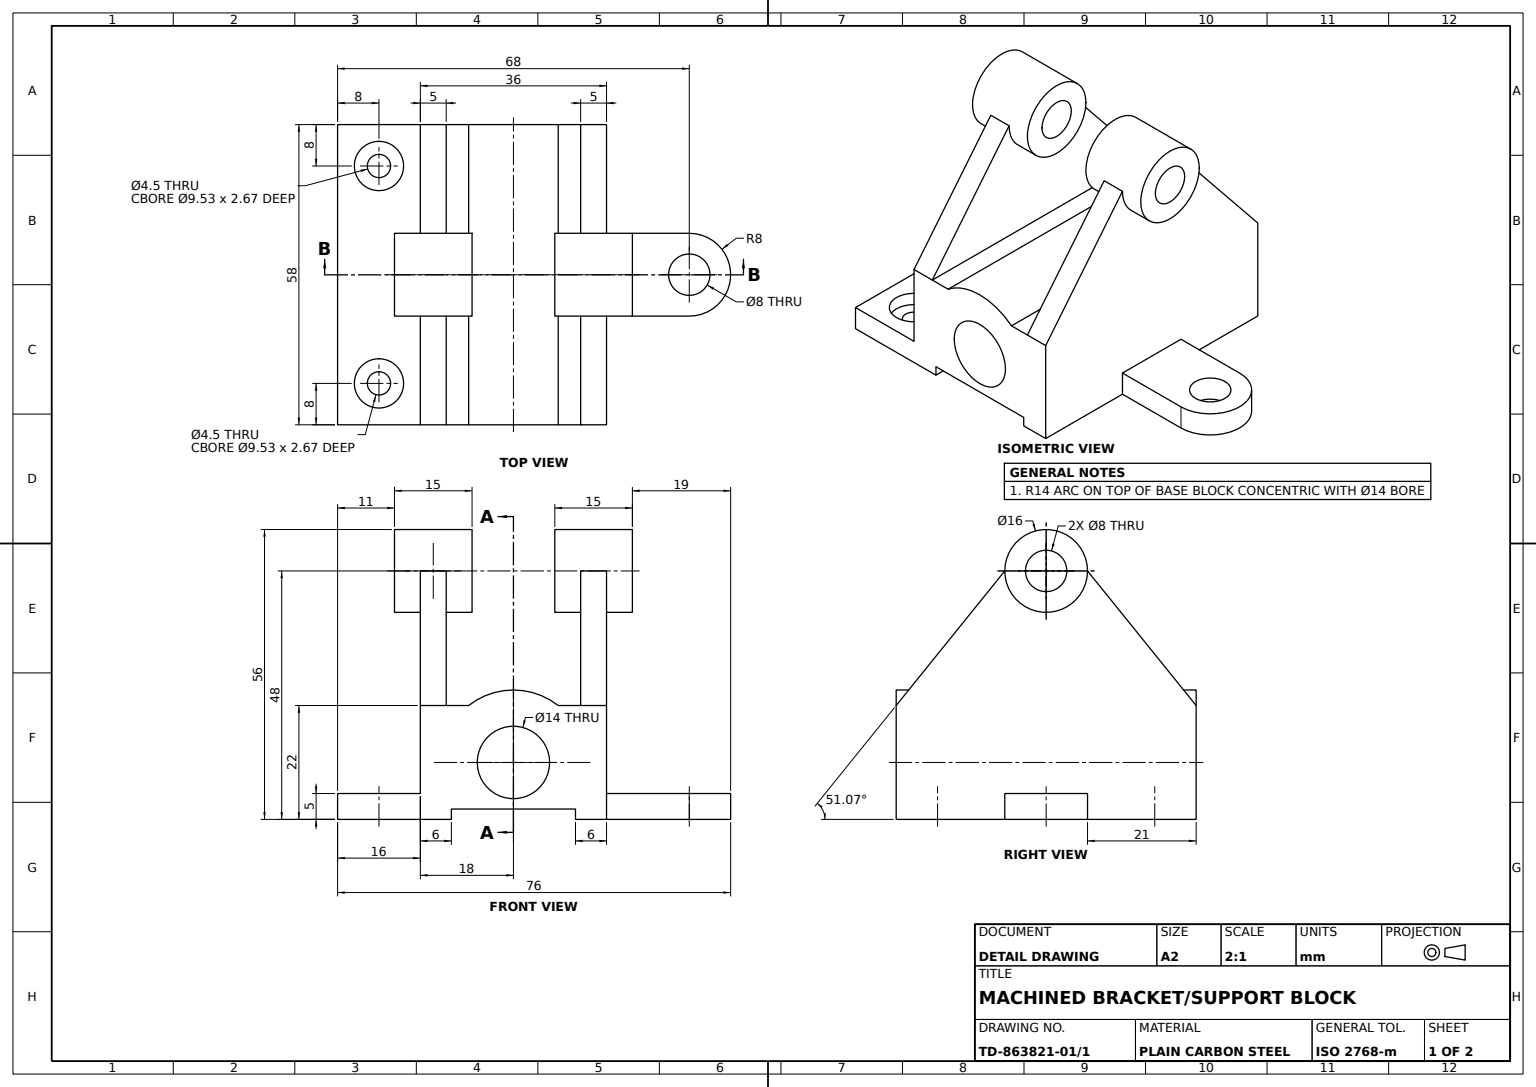
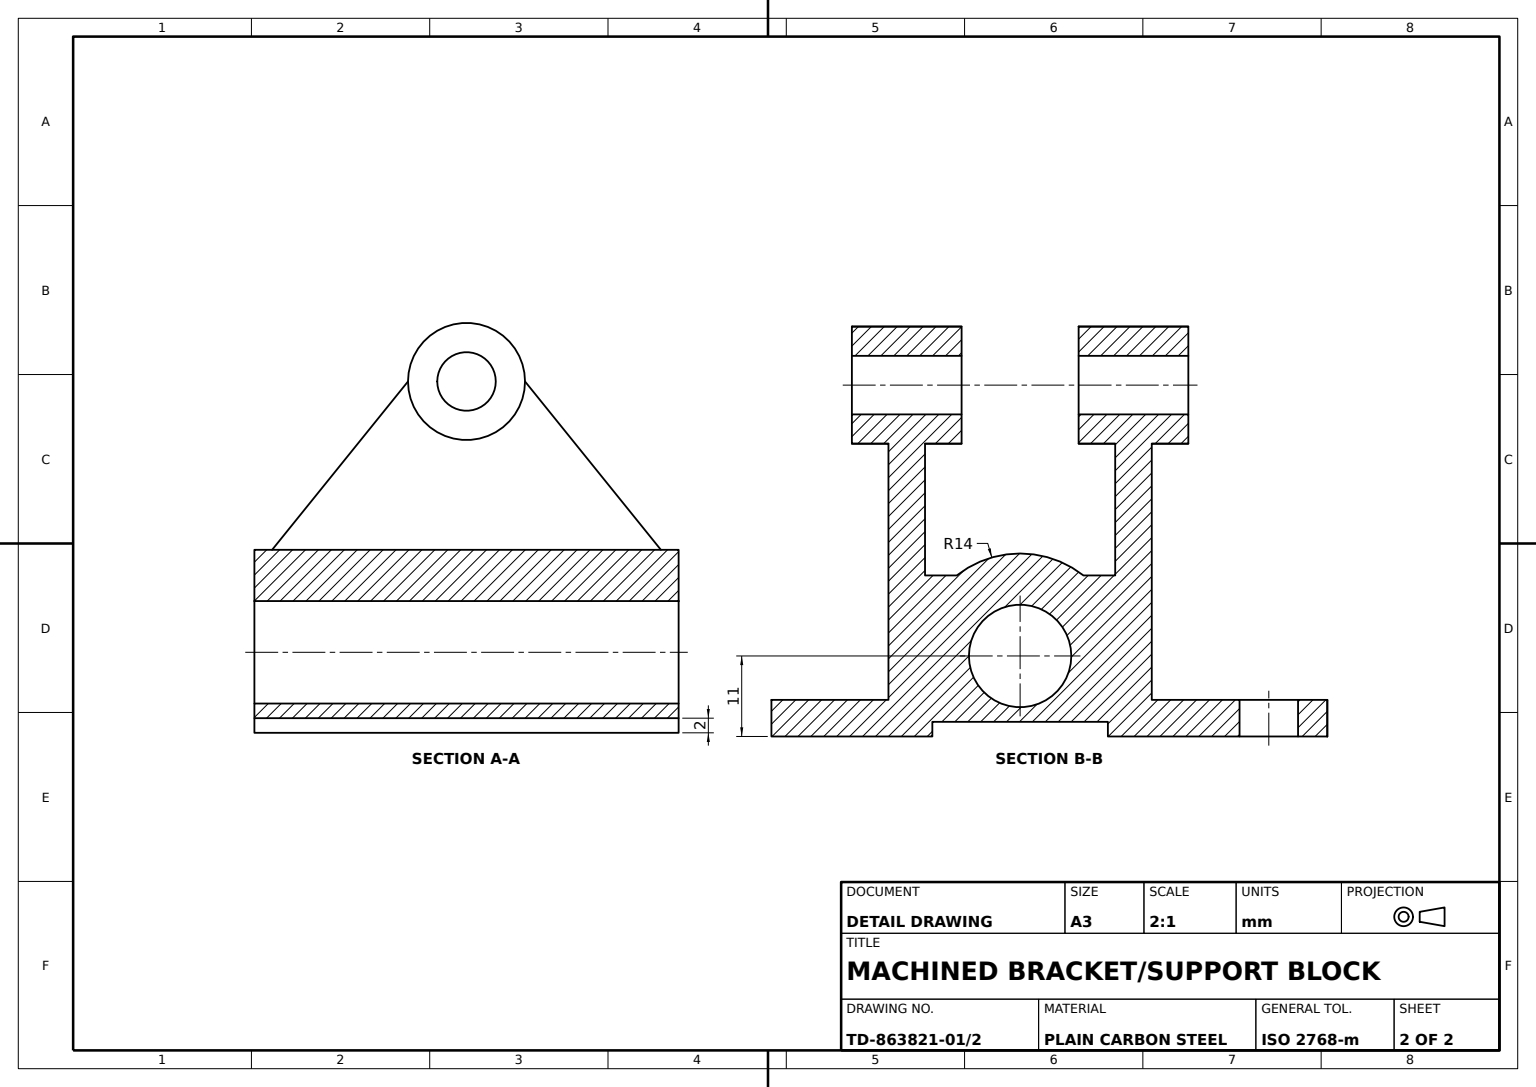
ISO-10303-21;
HEADER;
FILE_DESCRIPTION((''),'2;1');
FILE_NAME('','',(''),(''),'','','');
FILE_SCHEMA(('AUTOMOTIVE_DESIGN'));
ENDSEC;
DATA;
#1=APPLICATION_CONTEXT('');
#2=PRODUCT_CONTEXT('',#1,'mechanical');
#3=PRODUCT('','','',(#2));
#4=PRODUCT_DEFINITION_FORMATION('','',#3);
#5=PRODUCT_DEFINITION_CONTEXT('',#1,'design');
#6=PRODUCT_DEFINITION('','',#4,#5);
#7=PRODUCT_DEFINITION_SHAPE('','',#6);
#8=(LENGTH_UNIT()NAMED_UNIT(*)SI_UNIT(.MILLI.,.METRE.));
#9=(NAMED_UNIT(*)PLANE_ANGLE_UNIT()SI_UNIT($,.RADIAN.));
#10=(NAMED_UNIT(*)SI_UNIT($,.STERADIAN.)SOLID_ANGLE_UNIT());
#11=UNCERTAINTY_MEASURE_WITH_UNIT(LENGTH_MEASURE(1.E-05),#8,'distance_accuracy_value','');
#12=(GEOMETRIC_REPRESENTATION_CONTEXT(3)GLOBAL_UNCERTAINTY_ASSIGNED_CONTEXT((#11))GLOBAL_UNIT_ASSIGNED_CONTEXT((#8,#9,#10))REPRESENTATION_CONTEXT('',''));
#13=CARTESIAN_POINT('',(-8.,0.,5.75));
#14=VERTEX_POINT('',#13);
#15=CARTESIAN_POINT('',(-8.,0.,10.25));
#16=VERTEX_POINT('',#15);
#17=CARTESIAN_POINT('',(-8.,0.,8.));
#18=DIRECTION('',(0.,1.,0.));
#19=DIRECTION('',(0.,0.,1.));
#20=AXIS2_PLACEMENT_3D('',#17,#18,#19);
#21=CIRCLE('',#20,2.25);
#22=EDGE_CURVE('',#14,#16,#21,.T.);
#23=ORIENTED_EDGE('',*,*,#22,.T.);
#24=EDGE_CURVE('',#16,#14,#21,.T.);
#25=ORIENTED_EDGE('',*,*,#24,.T.);
#26=EDGE_LOOP('',(#23,#25));
#27=FACE_BOUND('',#26,.T.);
#28=CARTESIAN_POINT('',(-16.,0.,0.));
#29=VERTEX_POINT('',#28);
#30=CARTESIAN_POINT('',(6.,0.,0.));
#31=VERTEX_POINT('',#30);
#32=CARTESIAN_POINT('',(0.,0.,0.));
#33=DIRECTION('',(1.,0.,0.));
#34=VECTOR('',#33,1000.);
#35=LINE('',#32,#34);
#36=EDGE_CURVE('',#29,#31,#35,.T.);
#37=ORIENTED_EDGE('',*,*,#36,.T.);
#38=CARTESIAN_POINT('',(6.,0.,58.));
#39=VERTEX_POINT('',#38);
#40=DIRECTION('',(0.,0.,-1.));
#41=VECTOR('',#40,1000.);
#42=LINE('',#38,#41);
#43=EDGE_CURVE('',#39,#31,#42,.T.);
#44=ORIENTED_EDGE('',*,*,#43,.F.);
#45=CARTESIAN_POINT('',(-16.,0.,58.));
#46=VERTEX_POINT('',#45);
#47=CARTESIAN_POINT('',(0.,0.,58.));
#48=LINE('',#47,#34);
#49=EDGE_CURVE('',#46,#39,#48,.T.);
#50=ORIENTED_EDGE('',*,*,#49,.F.);
#51=VECTOR('',#19,1000.);
#52=LINE('',#28,#51);
#53=EDGE_CURVE('',#29,#46,#52,.T.);
#54=ORIENTED_EDGE('',*,*,#53,.F.);
#55=EDGE_LOOP('',(#37,#44,#50,#54));
#56=FACE_OUTER_BOUND('',#55,.T.);
#57=CARTESIAN_POINT('',(-8.,0.,47.75));
#58=VERTEX_POINT('',#57);
#59=CARTESIAN_POINT('',(-8.,0.,52.25));
#60=VERTEX_POINT('',#59);
#61=CARTESIAN_POINT('',(-8.,0.,50.));
#62=AXIS2_PLACEMENT_3D('',#61,#18,#19);
#63=CIRCLE('',#62,2.25);
#64=EDGE_CURVE('',#58,#60,#63,.T.);
#65=ORIENTED_EDGE('',*,*,#64,.T.);
#66=EDGE_CURVE('',#60,#58,#63,.T.);
#67=ORIENTED_EDGE('',*,*,#66,.T.);
#68=EDGE_LOOP('',(#65,#67));
#69=FACE_BOUND('',#68,.T.);
#70=AXIS2_PLACEMENT_3D('',#47,#18,#19);
#71=PLANE('',#70);
#72=ADVANCED_FACE('',(#27,#56,#69),#71,.F.);
#73=CARTESIAN_POINT('',(52.,0.,25.));
#74=VERTEX_POINT('',#73);
#75=CARTESIAN_POINT('',(52.,0.,33.));
#76=VERTEX_POINT('',#75);
#77=CARTESIAN_POINT('',(52.,0.,29.));
#78=AXIS2_PLACEMENT_3D('',#77,#18,#19);
#79=CIRCLE('',#78,4.);
#80=EDGE_CURVE('',#74,#76,#79,.T.);
#81=ORIENTED_EDGE('',*,*,#80,.T.);
#82=EDGE_CURVE('',#76,#74,#79,.T.);
#83=ORIENTED_EDGE('',*,*,#82,.T.);
#84=EDGE_LOOP('',(#81,#83));
#85=FACE_BOUND('',#84,.T.);
#86=CARTESIAN_POINT('',(36.,0.,58.));
#87=VERTEX_POINT('',#86);
#88=CARTESIAN_POINT('',(36.,0.,37.));
#89=VERTEX_POINT('',#88);
#90=LINE('',#86,#41);
#91=EDGE_CURVE('',#87,#89,#90,.T.);
#92=ORIENTED_EDGE('',*,*,#91,.F.);
#93=CARTESIAN_POINT('',(30.,0.,58.));
#94=VERTEX_POINT('',#93);
#95=LINE('',#93,#34);
#96=EDGE_CURVE('',#94,#87,#95,.T.);
#97=ORIENTED_EDGE('',*,*,#96,.F.);
#98=CARTESIAN_POINT('',(30.,0.,0.));
#99=VERTEX_POINT('',#98);
#100=LINE('',#93,#41);
#101=EDGE_CURVE('',#94,#99,#100,.T.);
#102=ORIENTED_EDGE('',*,*,#101,.T.);
#103=CARTESIAN_POINT('',(36.,0.,0.));
#104=VERTEX_POINT('',#103);
#105=LINE('',#98,#34);
#106=EDGE_CURVE('',#99,#104,#105,.T.);
#107=ORIENTED_EDGE('',*,*,#106,.T.);
#108=CARTESIAN_POINT('',(36.,0.,21.));
#109=VERTEX_POINT('',#108);
#110=EDGE_CURVE('',#109,#104,#90,.T.);
#111=ORIENTED_EDGE('',*,*,#110,.F.);
#112=CARTESIAN_POINT('',(52.,0.,21.));
#113=VERTEX_POINT('',#112);
#114=DIRECTION('',(-1.,0.,0.));
#115=VECTOR('',#114,1000.);
#116=LINE('',#112,#115);
#117=EDGE_CURVE('',#113,#109,#116,.T.);
#118=ORIENTED_EDGE('',*,*,#117,.F.);
#119=CARTESIAN_POINT('',(52.,0.,37.));
#120=VERTEX_POINT('',#119);
#121=CIRCLE('',#78,8.);
#122=EDGE_CURVE('',#120,#113,#121,.T.);
#123=ORIENTED_EDGE('',*,*,#122,.F.);
#124=LINE('',#119,#34);
#125=EDGE_CURVE('',#89,#120,#124,.T.);
#126=ORIENTED_EDGE('',*,*,#125,.F.);
#127=EDGE_LOOP('',(#92,#97,#102,#107,#111,#118,#123,#126));
#128=FACE_OUTER_BOUND('',#127,.T.);
#129=AXIS2_PLACEMENT_3D('',#93,#18,#19);
#130=PLANE('',#129);
#131=ADVANCED_FACE('',(#85,#128),#130,.F.);
#132=CARTESIAN_POINT('',(9.339746,22.,0.));
#133=VERTEX_POINT('',#132);
#134=CARTESIAN_POINT('',(5.,22.,0.));
#135=VERTEX_POINT('',#134);
#136=CARTESIAN_POINT('',(36.,22.,0.));
#137=LINE('',#136,#115);
#138=EDGE_CURVE('',#133,#135,#137,.T.);
#139=ORIENTED_EDGE('',*,*,#138,.T.);
#140=CARTESIAN_POINT('',(5.,22.,58.));
#141=VERTEX_POINT('',#140);
#142=LINE('',#134,#41);
#143=EDGE_CURVE('',#141,#135,#142,.T.);
#144=ORIENTED_EDGE('',*,*,#143,.F.);
#145=CARTESIAN_POINT('',(9.339746,22.,58.));
#146=VERTEX_POINT('',#145);
#147=CARTESIAN_POINT('',(36.,22.,58.));
#148=LINE('',#147,#115);
#149=EDGE_CURVE('',#146,#141,#148,.T.);
#150=ORIENTED_EDGE('',*,*,#149,.F.);
#151=LINE('',#132,#41);
#152=EDGE_CURVE('',#146,#133,#151,.T.);
#153=ORIENTED_EDGE('',*,*,#152,.T.);
#154=EDGE_LOOP('',(#139,#144,#150,#153));
#155=FACE_OUTER_BOUND('',#154,.T.);
#156=DIRECTION('',(0.,-1.,0.));
#157=AXIS2_PLACEMENT_3D('',#147,#156,#33);
#158=PLANE('',#157);
#159=ADVANCED_FACE('',(#155),#158,.F.);
#160=CARTESIAN_POINT('',(31.,22.,58.));
#161=VERTEX_POINT('',#160);
#162=CARTESIAN_POINT('',(26.660254,22.,58.));
#163=VERTEX_POINT('',#162);
#164=EDGE_CURVE('',#161,#163,#148,.T.);
#165=ORIENTED_EDGE('',*,*,#164,.F.);
#166=CARTESIAN_POINT('',(31.,22.,0.));
#167=VERTEX_POINT('',#166);
#168=LINE('',#160,#41);
#169=EDGE_CURVE('',#161,#167,#168,.T.);
#170=ORIENTED_EDGE('',*,*,#169,.T.);
#171=CARTESIAN_POINT('',(26.660254,22.,0.));
#172=VERTEX_POINT('',#171);
#173=EDGE_CURVE('',#167,#172,#137,.T.);
#174=ORIENTED_EDGE('',*,*,#173,.T.);
#175=LINE('',#171,#51);
#176=EDGE_CURVE('',#172,#163,#175,.T.);
#177=ORIENTED_EDGE('',*,*,#176,.T.);
#178=EDGE_LOOP('',(#165,#170,#174,#177));
#179=FACE_OUTER_BOUND('',#178,.T.);
#180=ADVANCED_FACE('',(#179),#158,.F.);
#181=CARTESIAN_POINT('',(41.,48.,25.));
#182=VERTEX_POINT('',#181);
#183=CARTESIAN_POINT('',(26.,48.,25.));
#184=VERTEX_POINT('',#183);
#185=LINE('',#181,#115);
#186=EDGE_CURVE('',#182,#184,#185,.T.);
#187=ORIENTED_EDGE('',*,*,#186,.T.);
#188=CARTESIAN_POINT('',(26.,48.,33.));
#189=VERTEX_POINT('',#188);
#190=CARTESIAN_POINT('',(26.,48.,29.));
#191=AXIS2_PLACEMENT_3D('',#190,#114,#19);
#192=CIRCLE('',#191,4.);
#193=EDGE_CURVE('',#184,#189,#192,.T.);
#194=ORIENTED_EDGE('',*,*,#193,.T.);
#195=CARTESIAN_POINT('',(41.,48.,33.));
#196=VERTEX_POINT('',#195);
#197=LINE('',#195,#115);
#198=EDGE_CURVE('',#196,#189,#197,.T.);
#199=ORIENTED_EDGE('',*,*,#198,.F.);
#200=CARTESIAN_POINT('',(41.,48.,29.));
#201=AXIS2_PLACEMENT_3D('',#200,#33,#40);
#202=CIRCLE('',#201,4.);
#203=EDGE_CURVE('',#196,#182,#202,.T.);
#204=ORIENTED_EDGE('',*,*,#203,.T.);
#205=EDGE_LOOP('',(#187,#194,#199,#204));
#206=FACE_OUTER_BOUND('',#205,.T.);
#207=AXIS2_PLACEMENT_3D('',#200,#114,#19);
#208=CYLINDRICAL_SURFACE('',#207,4.);
#209=ADVANCED_FACE('',(#206),#208,.F.);
#210=CARTESIAN_POINT('',(52.,5.,21.));
#211=VERTEX_POINT('',#210);
#212=CARTESIAN_POINT('',(36.,5.,21.));
#213=VERTEX_POINT('',#212);
#214=LINE('',#210,#115);
#215=EDGE_CURVE('',#211,#213,#214,.T.);
#216=ORIENTED_EDGE('',*,*,#215,.T.);
#217=CARTESIAN_POINT('',(36.,5.,37.));
#218=VERTEX_POINT('',#217);
#219=LINE('',#217,#51);
#220=EDGE_CURVE('',#213,#218,#219,.T.);
#221=ORIENTED_EDGE('',*,*,#220,.T.);
#222=CARTESIAN_POINT('',(52.,5.,37.));
#223=VERTEX_POINT('',#222);
#224=LINE('',#222,#34);
#225=EDGE_CURVE('',#218,#223,#224,.T.);
#226=ORIENTED_EDGE('',*,*,#225,.T.);
#227=CARTESIAN_POINT('',(52.,5.,29.));
#228=AXIS2_PLACEMENT_3D('',#227,#18,#19);
#229=CIRCLE('',#228,8.);
#230=EDGE_CURVE('',#223,#211,#229,.T.);
#231=ORIENTED_EDGE('',*,*,#230,.T.);
#232=EDGE_LOOP('',(#216,#221,#226,#231));
#233=FACE_OUTER_BOUND('',#232,.T.);
#234=CARTESIAN_POINT('',(52.,5.,33.));
#235=VERTEX_POINT('',#234);
#236=CARTESIAN_POINT('',(52.,5.,25.));
#237=VERTEX_POINT('',#236);
#238=CIRCLE('',#228,4.);
#239=EDGE_CURVE('',#235,#237,#238,.T.);
#240=ORIENTED_EDGE('',*,*,#239,.F.);
#241=EDGE_CURVE('',#237,#235,#238,.T.);
#242=ORIENTED_EDGE('',*,*,#241,.F.);
#243=EDGE_LOOP('',(#240,#242));
#244=FACE_BOUND('',#243,.T.);
#245=PLANE('',#228);
#246=ADVANCED_FACE('',(#233,#244),#245,.T.);
#247=CARTESIAN_POINT('',(10.,48.,33.));
#248=VERTEX_POINT('',#247);
#249=CARTESIAN_POINT('',(-5.,48.,33.));
#250=VERTEX_POINT('',#249);
#251=CARTESIAN_POINT('',(5.,48.,33.));
#252=LINE('',#251,#115);
#253=EDGE_CURVE('',#248,#250,#252,.T.);
#254=ORIENTED_EDGE('',*,*,#253,.F.);
#255=CARTESIAN_POINT('',(10.,48.,25.));
#256=VERTEX_POINT('',#255);
#257=CARTESIAN_POINT('',(10.,48.,29.));
#258=AXIS2_PLACEMENT_3D('',#257,#33,#40);
#259=CIRCLE('',#258,4.);
#260=EDGE_CURVE('',#248,#256,#259,.T.);
#261=ORIENTED_EDGE('',*,*,#260,.T.);
#262=CARTESIAN_POINT('',(-5.,48.,25.));
#263=VERTEX_POINT('',#262);
#264=CARTESIAN_POINT('',(5.,48.,25.));
#265=LINE('',#264,#115);
#266=EDGE_CURVE('',#256,#263,#265,.T.);
#267=ORIENTED_EDGE('',*,*,#266,.T.);
#268=CARTESIAN_POINT('',(-5.,48.,29.));
#269=AXIS2_PLACEMENT_3D('',#268,#33,#40);
#270=CIRCLE('',#269,4.);
#271=EDGE_CURVE('',#250,#263,#270,.T.);
#272=ORIENTED_EDGE('',*,*,#271,.F.);
#273=EDGE_LOOP('',(#254,#261,#267,#272));
#274=FACE_OUTER_BOUND('',#273,.T.);
#275=CARTESIAN_POINT('',(5.,48.,29.));
#276=AXIS2_PLACEMENT_3D('',#275,#114,#19);
#277=CYLINDRICAL_SURFACE('',#276,4.);
#278=ADVANCED_FACE('',(#274),#277,.F.);
#279=ORIENTED_EDGE('',*,*,#176,.F.);
#280=CARTESIAN_POINT('',(18.,11.,0.));
#281=AXIS2_PLACEMENT_3D('',#280,#19,#33);
#282=CIRCLE('',#281,14.);
#283=EDGE_CURVE('',#172,#133,#282,.T.);
#284=ORIENTED_EDGE('',*,*,#283,.T.);
#285=ORIENTED_EDGE('',*,*,#152,.F.);
#286=CARTESIAN_POINT('',(18.,11.,58.));
#287=AXIS2_PLACEMENT_3D('',#286,#19,#33);
#288=CIRCLE('',#287,14.);
#289=EDGE_CURVE('',#163,#146,#288,.T.);
#290=ORIENTED_EDGE('',*,*,#289,.F.);
#291=EDGE_LOOP('',(#279,#284,#285,#290));
#292=FACE_OUTER_BOUND('',#291,.T.);
#293=CYLINDRICAL_SURFACE('',#281,14.);
#294=ADVANCED_FACE('',(#292),#293,.T.);
#295=CARTESIAN_POINT('',(-8.,2.33,52.25));
#296=VERTEX_POINT('',#295);
#297=CARTESIAN_POINT('',(-8.,2.33,47.75));
#298=VERTEX_POINT('',#297);
#299=CARTESIAN_POINT('',(-8.,2.33,50.));
#300=AXIS2_PLACEMENT_3D('',#299,#18,#19);
#301=CIRCLE('',#300,2.25);
#302=EDGE_CURVE('',#296,#298,#301,.T.);
#303=ORIENTED_EDGE('',*,*,#302,.T.);
#304=CARTESIAN_POINT('',(-8.,5.,47.75));
#305=VECTOR('',#18,1000.);
#306=LINE('',#304,#305);
#307=EDGE_CURVE('',#58,#298,#306,.T.);
#308=ORIENTED_EDGE('',*,*,#307,.F.);
#309=ORIENTED_EDGE('',*,*,#66,.F.);
#310=CARTESIAN_POINT('',(-8.,5.,52.25));
#311=LINE('',#310,#305);
#312=EDGE_CURVE('',#60,#296,#311,.T.);
#313=ORIENTED_EDGE('',*,*,#312,.T.);
#314=EDGE_LOOP('',(#303,#308,#309,#313));
#315=FACE_OUTER_BOUND('',#314,.T.);
#316=CARTESIAN_POINT('',(-8.,5.,50.));
#317=AXIS2_PLACEMENT_3D('',#316,#18,#19);
#318=CYLINDRICAL_SURFACE('',#317,2.25);
#319=ADVANCED_FACE('',(#315),#318,.F.);
#320=CARTESIAN_POINT('',(-8.,2.33,5.75));
#321=VERTEX_POINT('',#320);
#322=CARTESIAN_POINT('',(-8.,5.,5.75));
#323=LINE('',#322,#305);
#324=EDGE_CURVE('',#14,#321,#323,.T.);
#325=ORIENTED_EDGE('',*,*,#324,.T.);
#326=CARTESIAN_POINT('',(-8.,2.33,10.25));
#327=VERTEX_POINT('',#326);
#328=CARTESIAN_POINT('',(-8.,2.33,8.));
#329=AXIS2_PLACEMENT_3D('',#328,#18,#19);
#330=CIRCLE('',#329,2.25);
#331=EDGE_CURVE('',#321,#327,#330,.T.);
#332=ORIENTED_EDGE('',*,*,#331,.T.);
#333=CARTESIAN_POINT('',(-8.,5.,10.25));
#334=LINE('',#333,#305);
#335=EDGE_CURVE('',#16,#327,#334,.T.);
#336=ORIENTED_EDGE('',*,*,#335,.F.);
#337=ORIENTED_EDGE('',*,*,#22,.F.);
#338=EDGE_LOOP('',(#325,#332,#336,#337));
#339=FACE_OUTER_BOUND('',#338,.T.);
#340=CARTESIAN_POINT('',(-8.,5.,8.));
#341=AXIS2_PLACEMENT_3D('',#340,#18,#19);
#342=CYLINDRICAL_SURFACE('',#341,2.25);
#343=ADVANCED_FACE('',(#339),#342,.F.);
#344=CARTESIAN_POINT('',(-8.,5.,12.765));
#345=VERTEX_POINT('',#344);
#346=CARTESIAN_POINT('',(-8.,5.,3.235));
#347=VERTEX_POINT('',#346);
#348=CIRCLE('',#341,4.765);
#349=EDGE_CURVE('',#345,#347,#348,.T.);
#350=ORIENTED_EDGE('',*,*,#349,.T.);
#351=CARTESIAN_POINT('',(-8.,2.33,3.235));
#352=VERTEX_POINT('',#351);
#353=LINE('',#346,#305);
#354=EDGE_CURVE('',#352,#347,#353,.T.);
#355=ORIENTED_EDGE('',*,*,#354,.F.);
#356=CARTESIAN_POINT('',(-8.,2.33,12.765));
#357=VERTEX_POINT('',#356);
#358=CIRCLE('',#329,4.765);
#359=EDGE_CURVE('',#357,#352,#358,.T.);
#360=ORIENTED_EDGE('',*,*,#359,.F.);
#361=LINE('',#344,#305);
#362=EDGE_CURVE('',#357,#345,#361,.T.);
#363=ORIENTED_EDGE('',*,*,#362,.T.);
#364=EDGE_LOOP('',(#350,#355,#360,#363));
#365=FACE_OUTER_BOUND('',#364,.T.);
#366=CYLINDRICAL_SURFACE('',#341,4.765);
#367=ADVANCED_FACE('',(#365),#366,.F.);
#368=CARTESIAN_POINT('',(11.,11.,0.));
#369=VERTEX_POINT('',#368);
#370=CARTESIAN_POINT('',(11.,11.,58.));
#371=VERTEX_POINT('',#370);
#372=LINE('',#368,#51);
#373=EDGE_CURVE('',#369,#371,#372,.T.);
#374=ORIENTED_EDGE('',*,*,#373,.F.);
#375=CARTESIAN_POINT('',(25.,11.,0.));
#376=VERTEX_POINT('',#375);
#377=CIRCLE('',#281,7.);
#378=EDGE_CURVE('',#376,#369,#377,.T.);
#379=ORIENTED_EDGE('',*,*,#378,.F.);
#380=CARTESIAN_POINT('',(25.,11.,58.));
#381=VERTEX_POINT('',#380);
#382=LINE('',#375,#51);
#383=EDGE_CURVE('',#376,#381,#382,.T.);
#384=ORIENTED_EDGE('',*,*,#383,.T.);
#385=CIRCLE('',#287,7.);
#386=EDGE_CURVE('',#381,#371,#385,.T.);
#387=ORIENTED_EDGE('',*,*,#386,.T.);
#388=EDGE_LOOP('',(#374,#379,#384,#387));
#389=FACE_OUTER_BOUND('',#388,.T.);
#390=CYLINDRICAL_SURFACE('',#281,7.);
#391=ADVANCED_FACE('',(#389),#390,.F.);
#392=CARTESIAN_POINT('',(36.,48.,21.));
#393=VERTEX_POINT('',#392);
#394=CARTESIAN_POINT('',(36.,48.,37.));
#395=VERTEX_POINT('',#394);
#396=CARTESIAN_POINT('',(36.,48.,29.));
#397=AXIS2_PLACEMENT_3D('',#396,#114,#40);
#398=CIRCLE('',#397,8.);
#399=EDGE_CURVE('',#393,#395,#398,.T.);
#400=ORIENTED_EDGE('',*,*,#399,.F.);
#401=CARTESIAN_POINT('',(41.,48.,21.));
#402=VERTEX_POINT('',#401);
#403=LINE('',#401,#115);
#404=EDGE_CURVE('',#402,#393,#403,.T.);
#405=ORIENTED_EDGE('',*,*,#404,.F.);
#406=CARTESIAN_POINT('',(41.,48.,37.));
#407=VERTEX_POINT('',#406);
#408=CIRCLE('',#201,8.);
#409=EDGE_CURVE('',#407,#402,#408,.T.);
#410=ORIENTED_EDGE('',*,*,#409,.F.);
#411=LINE('',#406,#115);
#412=EDGE_CURVE('',#407,#395,#411,.T.);
#413=ORIENTED_EDGE('',*,*,#412,.T.);
#414=EDGE_LOOP('',(#400,#405,#410,#413));
#415=FACE_OUTER_BOUND('',#414,.T.);
#416=CYLINDRICAL_SURFACE('',#207,8.);
#417=ADVANCED_FACE('',(#415),#416,.T.);
#418=CARTESIAN_POINT('',(26.,48.,21.));
#419=VERTEX_POINT('',#418);
#420=CARTESIAN_POINT('',(26.,48.,37.));
#421=VERTEX_POINT('',#420);
#422=CIRCLE('',#191,8.);
#423=EDGE_CURVE('',#419,#421,#422,.T.);
#424=ORIENTED_EDGE('',*,*,#423,.F.);
#425=CARTESIAN_POINT('',(31.,48.,21.));
#426=VERTEX_POINT('',#425);
#427=EDGE_CURVE('',#426,#419,#403,.T.);
#428=ORIENTED_EDGE('',*,*,#427,.F.);
#429=CARTESIAN_POINT('',(31.,48.,37.));
#430=VERTEX_POINT('',#429);
#431=CARTESIAN_POINT('',(31.,48.,29.));
#432=AXIS2_PLACEMENT_3D('',#431,#114,#19);
#433=CIRCLE('',#432,8.);
#434=EDGE_CURVE('',#426,#430,#433,.T.);
#435=ORIENTED_EDGE('',*,*,#434,.T.);
#436=EDGE_CURVE('',#430,#421,#411,.T.);
#437=ORIENTED_EDGE('',*,*,#436,.T.);
#438=EDGE_LOOP('',(#424,#428,#435,#437));
#439=FACE_OUTER_BOUND('',#438,.T.);
#440=ADVANCED_FACE('',(#439),#416,.T.);
#441=CARTESIAN_POINT('',(0.,5.,58.));
#442=VERTEX_POINT('',#441);
#443=CARTESIAN_POINT('',(0.,5.,0.));
#444=VERTEX_POINT('',#443);
#445=LINE('',#441,#41);
#446=EDGE_CURVE('',#442,#444,#445,.T.);
#447=ORIENTED_EDGE('',*,*,#446,.F.);
#448=CARTESIAN_POINT('',(0.,22.,58.));
#449=VERTEX_POINT('',#448);
#450=VECTOR('',#156,1000.);
#451=LINE('',#448,#450);
#452=EDGE_CURVE('',#449,#442,#451,.T.);
#453=ORIENTED_EDGE('',*,*,#452,.F.);
#454=CARTESIAN_POINT('',(0.,48.,37.));
#455=VERTEX_POINT('',#454);
#456=DIRECTION('',(0.,-0.77794118,0.628337107));
#457=VECTOR('',#456,1000.);
#458=LINE('',#448,#457);
#459=EDGE_CURVE('',#455,#449,#458,.T.);
#460=ORIENTED_EDGE('',*,*,#459,.F.);
#461=CARTESIAN_POINT('',(0.,48.,21.));
#462=VERTEX_POINT('',#461);
#463=CARTESIAN_POINT('',(0.,48.,29.));
#464=AXIS2_PLACEMENT_3D('',#463,#114,#19);
#465=CIRCLE('',#464,8.);
#466=EDGE_CURVE('',#462,#455,#465,.T.);
#467=ORIENTED_EDGE('',*,*,#466,.F.);
#468=CARTESIAN_POINT('',(0.,22.,0.));
#469=VERTEX_POINT('',#468);
#470=DIRECTION('',(0.,0.77794118,0.628337107));
#471=VECTOR('',#470,1000.);
#472=LINE('',#461,#471);
#473=EDGE_CURVE('',#469,#462,#472,.T.);
#474=ORIENTED_EDGE('',*,*,#473,.F.);
#475=LINE('',#468,#450);
#476=EDGE_CURVE('',#469,#444,#475,.T.);
#477=ORIENTED_EDGE('',*,*,#476,.T.);
#478=EDGE_LOOP('',(#447,#453,#460,#467,#474,#477));
#479=FACE_OUTER_BOUND('',#478,.T.);
#480=AXIS2_PLACEMENT_3D('',#448,#33,#18);
#481=PLANE('',#480);
#482=ADVANCED_FACE('',(#479),#481,.F.);
#483=LINE('',#236,#450);
#484=EDGE_CURVE('',#237,#74,#483,.T.);
#485=ORIENTED_EDGE('',*,*,#484,.T.);
#486=ORIENTED_EDGE('',*,*,#82,.F.);
#487=LINE('',#234,#450);
#488=EDGE_CURVE('',#235,#76,#487,.T.);
#489=ORIENTED_EDGE('',*,*,#488,.F.);
#490=ORIENTED_EDGE('',*,*,#239,.T.);
#491=EDGE_LOOP('',(#485,#486,#489,#490));
#492=FACE_OUTER_BOUND('',#491,.T.);
#493=AXIS2_PLACEMENT_3D('',#227,#156,#40);
#494=CYLINDRICAL_SURFACE('',#493,4.);
#495=ADVANCED_FACE('',(#492),#494,.F.);
#496=CARTESIAN_POINT('',(10.,48.,21.));
#497=VERTEX_POINT('',#496);
#498=CARTESIAN_POINT('',(5.,48.,21.));
#499=VERTEX_POINT('',#498);
#500=LINE('',#498,#115);
#501=EDGE_CURVE('',#497,#499,#500,.T.);
#502=ORIENTED_EDGE('',*,*,#501,.F.);
#503=CARTESIAN_POINT('',(10.,48.,37.));
#504=VERTEX_POINT('',#503);
#505=CIRCLE('',#258,8.);
#506=EDGE_CURVE('',#504,#497,#505,.T.);
#507=ORIENTED_EDGE('',*,*,#506,.F.);
#508=CARTESIAN_POINT('',(5.,48.,37.));
#509=VERTEX_POINT('',#508);
#510=LINE('',#508,#115);
#511=EDGE_CURVE('',#504,#509,#510,.T.);
#512=ORIENTED_EDGE('',*,*,#511,.T.);
#513=AXIS2_PLACEMENT_3D('',#275,#33,#40);
#514=CIRCLE('',#513,8.);
#515=EDGE_CURVE('',#509,#499,#514,.T.);
#516=ORIENTED_EDGE('',*,*,#515,.T.);
#517=EDGE_LOOP('',(#502,#507,#512,#516));
#518=FACE_OUTER_BOUND('',#517,.T.);
#519=CYLINDRICAL_SURFACE('',#276,8.);
#520=ADVANCED_FACE('',(#518),#519,.T.);
#521=EDGE_CURVE('',#327,#321,#330,.T.);
#522=ORIENTED_EDGE('',*,*,#521,.T.);
#523=ORIENTED_EDGE('',*,*,#324,.F.);
#524=ORIENTED_EDGE('',*,*,#24,.F.);
#525=ORIENTED_EDGE('',*,*,#335,.T.);
#526=EDGE_LOOP('',(#522,#523,#524,#525));
#527=FACE_OUTER_BOUND('',#526,.T.);
#528=ADVANCED_FACE('',(#527),#342,.F.);
#529=CARTESIAN_POINT('',(-5.,48.,37.));
#530=VERTEX_POINT('',#529);
#531=EDGE_CURVE('',#455,#530,#510,.T.);
#532=ORIENTED_EDGE('',*,*,#531,.T.);
#533=CARTESIAN_POINT('',(-5.,48.,21.));
#534=VERTEX_POINT('',#533);
#535=CIRCLE('',#269,8.);
#536=EDGE_CURVE('',#530,#534,#535,.T.);
#537=ORIENTED_EDGE('',*,*,#536,.T.);
#538=EDGE_CURVE('',#462,#534,#500,.T.);
#539=ORIENTED_EDGE('',*,*,#538,.F.);
#540=ORIENTED_EDGE('',*,*,#466,.T.);
#541=EDGE_LOOP('',(#532,#537,#539,#540));
#542=FACE_OUTER_BOUND('',#541,.T.);
#543=ADVANCED_FACE('',(#542),#519,.T.);
#544=LINE('',#425,#34);
#545=EDGE_CURVE('',#426,#393,#544,.T.);
#546=ORIENTED_EDGE('',*,*,#545,.T.);
#547=VERTEX_POINT('',#136);
#548=LINE('',#136,#471);
#549=EDGE_CURVE('',#547,#393,#548,.T.);
#550=ORIENTED_EDGE('',*,*,#549,.F.);
#551=EDGE_CURVE('',#547,#167,#137,.T.);
#552=ORIENTED_EDGE('',*,*,#551,.T.);
#553=LINE('',#166,#471);
#554=EDGE_CURVE('',#167,#426,#553,.T.);
#555=ORIENTED_EDGE('',*,*,#554,.T.);
#556=EDGE_LOOP('',(#546,#550,#552,#555));
#557=FACE_OUTER_BOUND('',#556,.T.);
#558=DIRECTION('',(0.,0.628337107,-0.77794118));
#559=AXIS2_PLACEMENT_3D('',#166,#558,#470);
#560=PLANE('',#559);
#561=ADVANCED_FACE('',(#557),#560,.T.);
#562=CARTESIAN_POINT('',(-8.,2.33,54.765));
#563=VERTEX_POINT('',#562);
#564=CARTESIAN_POINT('',(-8.,2.33,45.235));
#565=VERTEX_POINT('',#564);
#566=CIRCLE('',#300,4.765);
#567=EDGE_CURVE('',#563,#565,#566,.T.);
#568=ORIENTED_EDGE('',*,*,#567,.T.);
#569=EDGE_CURVE('',#565,#563,#566,.T.);
#570=ORIENTED_EDGE('',*,*,#569,.T.);
#571=EDGE_LOOP('',(#568,#570));
#572=FACE_OUTER_BOUND('',#571,.T.);
#573=ORIENTED_EDGE('',*,*,#302,.F.);
#574=EDGE_CURVE('',#298,#296,#301,.T.);
#575=ORIENTED_EDGE('',*,*,#574,.F.);
#576=EDGE_LOOP('',(#573,#575));
#577=FACE_BOUND('',#576,.T.);
#578=CARTESIAN_POINT('',(-5.75,2.33,50.));
#579=AXIS2_PLACEMENT_3D('',#578,#156,#40);
#580=PLANE('',#579);
#581=ADVANCED_FACE('',(#572,#577),#580,.F.);
#582=ORIENTED_EDGE('',*,*,#362,.F.);
#583=EDGE_CURVE('',#352,#357,#358,.T.);
#584=ORIENTED_EDGE('',*,*,#583,.F.);
#585=ORIENTED_EDGE('',*,*,#354,.T.);
#586=EDGE_CURVE('',#347,#345,#348,.T.);
#587=ORIENTED_EDGE('',*,*,#586,.T.);
#588=EDGE_LOOP('',(#582,#584,#585,#587));
#589=FACE_OUTER_BOUND('',#588,.T.);
#590=ADVANCED_FACE('',(#589),#366,.F.);
#591=ORIENTED_EDGE('',*,*,#383,.F.);
#592=EDGE_CURVE('',#369,#376,#377,.T.);
#593=ORIENTED_EDGE('',*,*,#592,.F.);
#594=ORIENTED_EDGE('',*,*,#373,.T.);
#595=EDGE_CURVE('',#371,#381,#385,.T.);
#596=ORIENTED_EDGE('',*,*,#595,.T.);
#597=EDGE_LOOP('',(#591,#593,#594,#596));
#598=FACE_OUTER_BOUND('',#597,.T.);
#599=ADVANCED_FACE('',(#598),#390,.F.);
#600=LINE('',#140,#457);
#601=EDGE_CURVE('',#509,#141,#600,.T.);
#602=ORIENTED_EDGE('',*,*,#601,.T.);
#603=ORIENTED_EDGE('',*,*,#143,.T.);
#604=LINE('',#498,#471);
#605=EDGE_CURVE('',#135,#499,#604,.T.);
#606=ORIENTED_EDGE('',*,*,#605,.T.);
#607=ORIENTED_EDGE('',*,*,#515,.F.);
#608=EDGE_LOOP('',(#602,#603,#606,#607));
#609=FACE_OUTER_BOUND('',#608,.T.);
#610=PLANE('',#276);
#611=ADVANCED_FACE('',(#609),#610,.F.);
#612=CARTESIAN_POINT('',(6.,2.,58.));
#613=VERTEX_POINT('',#612);
#614=CARTESIAN_POINT('',(6.,2.,0.));
#615=VERTEX_POINT('',#614);
#616=LINE('',#612,#41);
#617=EDGE_CURVE('',#613,#615,#616,.T.);
#618=ORIENTED_EDGE('',*,*,#617,.F.);
#619=LINE('',#38,#305);
#620=EDGE_CURVE('',#39,#613,#619,.T.);
#621=ORIENTED_EDGE('',*,*,#620,.F.);
#622=ORIENTED_EDGE('',*,*,#43,.T.);
#623=LINE('',#30,#305);
#624=EDGE_CURVE('',#31,#615,#623,.T.);
#625=ORIENTED_EDGE('',*,*,#624,.T.);
#626=EDGE_LOOP('',(#618,#621,#622,#625));
#627=FACE_OUTER_BOUND('',#626,.T.);
#628=AXIS2_PLACEMENT_3D('',#38,#114,#19);
#629=PLANE('',#628);
#630=ADVANCED_FACE('',(#627),#629,.F.);
#631=ORIENTED_EDGE('',*,*,#359,.T.);
#632=ORIENTED_EDGE('',*,*,#583,.T.);
#633=EDGE_LOOP('',(#631,#632));
#634=FACE_OUTER_BOUND('',#633,.T.);
#635=ORIENTED_EDGE('',*,*,#521,.F.);
#636=ORIENTED_EDGE('',*,*,#331,.F.);
#637=EDGE_LOOP('',(#635,#636));
#638=FACE_BOUND('',#637,.T.);
#639=CARTESIAN_POINT('',(-5.75,2.33,8.));
#640=AXIS2_PLACEMENT_3D('',#639,#156,#40);
#641=PLANE('',#640);
#642=ADVANCED_FACE('',(#634,#638),#641,.F.);
#643=ORIENTED_EDGE('',*,*,#266,.F.);
#644=EDGE_CURVE('',#256,#248,#259,.T.);
#645=ORIENTED_EDGE('',*,*,#644,.T.);
#646=ORIENTED_EDGE('',*,*,#253,.T.);
#647=EDGE_CURVE('',#263,#250,#270,.T.);
#648=ORIENTED_EDGE('',*,*,#647,.F.);
#649=EDGE_LOOP('',(#643,#645,#646,#648));
#650=FACE_OUTER_BOUND('',#649,.T.);
#651=ADVANCED_FACE('',(#650),#277,.F.);
#652=ORIENTED_EDGE('',*,*,#586,.F.);
#653=ORIENTED_EDGE('',*,*,#349,.F.);
#654=EDGE_LOOP('',(#652,#653));
#655=FACE_BOUND('',#654,.T.);
#656=CARTESIAN_POINT('',(-8.,5.,45.235));
#657=VERTEX_POINT('',#656);
#658=CARTESIAN_POINT('',(-8.,5.,54.765));
#659=VERTEX_POINT('',#658);
#660=CIRCLE('',#317,4.765);
#661=EDGE_CURVE('',#657,#659,#660,.T.);
#662=ORIENTED_EDGE('',*,*,#661,.F.);
#663=EDGE_CURVE('',#659,#657,#660,.T.);
#664=ORIENTED_EDGE('',*,*,#663,.F.);
#665=EDGE_LOOP('',(#662,#664));
#666=FACE_BOUND('',#665,.T.);
#667=CARTESIAN_POINT('',(-16.,5.,0.));
#668=VERTEX_POINT('',#667);
#669=CARTESIAN_POINT('',(-16.,5.,58.));
#670=VERTEX_POINT('',#669);
#671=LINE('',#667,#51);
#672=EDGE_CURVE('',#668,#670,#671,.T.);
#673=ORIENTED_EDGE('',*,*,#672,.T.);
#674=LINE('',#669,#34);
#675=EDGE_CURVE('',#670,#442,#674,.T.);
#676=ORIENTED_EDGE('',*,*,#675,.T.);
#677=ORIENTED_EDGE('',*,*,#446,.T.);
#678=LINE('',#443,#115);
#679=EDGE_CURVE('',#444,#668,#678,.T.);
#680=ORIENTED_EDGE('',*,*,#679,.T.);
#681=EDGE_LOOP('',(#673,#676,#677,#680));
#682=FACE_OUTER_BOUND('',#681,.T.);
#683=AXIS2_PLACEMENT_3D('',#443,#18,#19);
#684=PLANE('',#683);
#685=ADVANCED_FACE('',(#655,#666,#682),#684,.T.);
#686=ORIENTED_EDGE('',*,*,#378,.T.);
#687=ORIENTED_EDGE('',*,*,#592,.T.);
#688=EDGE_LOOP('',(#686,#687));
#689=FACE_BOUND('',#688,.T.);
#690=ORIENTED_EDGE('',*,*,#476,.F.);
#691=LINE('',#134,#115);
#692=EDGE_CURVE('',#135,#469,#691,.T.);
#693=ORIENTED_EDGE('',*,*,#692,.F.);
#694=ORIENTED_EDGE('',*,*,#138,.F.);
#695=ORIENTED_EDGE('',*,*,#283,.F.);
#696=ORIENTED_EDGE('',*,*,#173,.F.);
#697=ORIENTED_EDGE('',*,*,#551,.F.);
#698=LINE('',#103,#305);
#699=EDGE_CURVE('',#104,#547,#698,.T.);
#700=ORIENTED_EDGE('',*,*,#699,.F.);
#701=ORIENTED_EDGE('',*,*,#106,.F.);
#702=CARTESIAN_POINT('',(30.,2.,0.));
#703=VERTEX_POINT('',#702);
#704=LINE('',#702,#450);
#705=EDGE_CURVE('',#703,#99,#704,.T.);
#706=ORIENTED_EDGE('',*,*,#705,.F.);
#707=LINE('',#614,#34);
#708=EDGE_CURVE('',#615,#703,#707,.T.);
#709=ORIENTED_EDGE('',*,*,#708,.F.);
#710=ORIENTED_EDGE('',*,*,#624,.F.);
#711=ORIENTED_EDGE('',*,*,#36,.F.);
#712=LINE('',#667,#450);
#713=EDGE_CURVE('',#668,#29,#712,.T.);
#714=ORIENTED_EDGE('',*,*,#713,.F.);
#715=ORIENTED_EDGE('',*,*,#679,.F.);
#716=EDGE_LOOP('',(#690,#693,#694,#695,#696,#697,#700,#701,#706,#709,#710,#711,#714,#715));
#717=FACE_OUTER_BOUND('',#716,.T.);
#718=AXIS2_PLACEMENT_3D('',#32,#19,#33);
#719=PLANE('',#718);
#720=ADVANCED_FACE('',(#689,#717),#719,.F.);
#721=LINE('',#429,#34);
#722=EDGE_CURVE('',#430,#395,#721,.T.);
#723=ORIENTED_EDGE('',*,*,#722,.F.);
#724=LINE('',#429,#457);
#725=EDGE_CURVE('',#430,#161,#724,.T.);
#726=ORIENTED_EDGE('',*,*,#725,.T.);
#727=VERTEX_POINT('',#147);
#728=EDGE_CURVE('',#727,#161,#148,.T.);
#729=ORIENTED_EDGE('',*,*,#728,.F.);
#730=LINE('',#394,#457);
#731=EDGE_CURVE('',#395,#727,#730,.T.);
#732=ORIENTED_EDGE('',*,*,#731,.F.);
#733=EDGE_LOOP('',(#723,#726,#729,#732));
#734=FACE_OUTER_BOUND('',#733,.T.);
#735=DIRECTION('',(0.,0.628337107,0.77794118));
#736=AXIS2_PLACEMENT_3D('',#429,#735,#456);
#737=PLANE('',#736);
#738=ADVANCED_FACE('',(#734),#737,.T.);
#739=ORIENTED_EDGE('',*,*,#722,.T.);
#740=ORIENTED_EDGE('',*,*,#412,.F.);
#741=EDGE_CURVE('',#402,#407,#408,.T.);
#742=ORIENTED_EDGE('',*,*,#741,.F.);
#743=ORIENTED_EDGE('',*,*,#404,.T.);
#744=ORIENTED_EDGE('',*,*,#545,.F.);
#745=ORIENTED_EDGE('',*,*,#427,.T.);
#746=EDGE_CURVE('',#421,#419,#422,.T.);
#747=ORIENTED_EDGE('',*,*,#746,.F.);
#748=ORIENTED_EDGE('',*,*,#436,.F.);
#749=EDGE_LOOP('',(#739,#740,#742,#743,#744,#745,#747,#748));
#750=FACE_OUTER_BOUND('',#749,.T.);
#751=ADVANCED_FACE('',(#750),#416,.T.);
#752=ORIENTED_EDGE('',*,*,#536,.F.);
#753=EDGE_CURVE('',#534,#530,#535,.T.);
#754=ORIENTED_EDGE('',*,*,#753,.F.);
#755=EDGE_LOOP('',(#752,#754));
#756=FACE_OUTER_BOUND('',#755,.T.);
#757=ORIENTED_EDGE('',*,*,#271,.T.);
#758=ORIENTED_EDGE('',*,*,#647,.T.);
#759=EDGE_LOOP('',(#757,#758));
#760=FACE_BOUND('',#759,.T.);
#761=PLANE('',#269);
#762=ADVANCED_FACE('',(#756,#760),#761,.F.);
#763=ORIENTED_EDGE('',*,*,#220,.F.);
#764=LINE('',#212,#450);
#765=EDGE_CURVE('',#213,#109,#764,.T.);
#766=ORIENTED_EDGE('',*,*,#765,.T.);
#767=ORIENTED_EDGE('',*,*,#110,.T.);
#768=ORIENTED_EDGE('',*,*,#699,.T.);
#769=ORIENTED_EDGE('',*,*,#549,.T.);
#770=ORIENTED_EDGE('',*,*,#399,.T.);
#771=ORIENTED_EDGE('',*,*,#731,.T.);
#772=LINE('',#86,#305);
#773=EDGE_CURVE('',#87,#727,#772,.T.);
#774=ORIENTED_EDGE('',*,*,#773,.F.);
#775=ORIENTED_EDGE('',*,*,#91,.T.);
#776=LINE('',#217,#450);
#777=EDGE_CURVE('',#218,#89,#776,.T.);
#778=ORIENTED_EDGE('',*,*,#777,.F.);
#779=EDGE_LOOP('',(#763,#766,#767,#768,#769,#770,#771,#774,#775,#778));
#780=FACE_OUTER_BOUND('',#779,.T.);
#781=AXIS2_PLACEMENT_3D('',#86,#114,#19);
#782=PLANE('',#781);
#783=ADVANCED_FACE('',(#780),#782,.F.);
#784=LINE('',#669,#450);
#785=EDGE_CURVE('',#670,#46,#784,.T.);
#786=ORIENTED_EDGE('',*,*,#785,.F.);
#787=ORIENTED_EDGE('',*,*,#672,.F.);
#788=ORIENTED_EDGE('',*,*,#713,.T.);
#789=ORIENTED_EDGE('',*,*,#53,.T.);
#790=EDGE_LOOP('',(#786,#787,#788,#789));
#791=FACE_OUTER_BOUND('',#790,.T.);
#792=AXIS2_PLACEMENT_3D('',#667,#33,#40);
#793=PLANE('',#792);
#794=ADVANCED_FACE('',(#791),#793,.F.);
#795=ORIENTED_EDGE('',*,*,#117,.T.);
#796=ORIENTED_EDGE('',*,*,#765,.F.);
#797=ORIENTED_EDGE('',*,*,#215,.F.);
#798=LINE('',#210,#450);
#799=EDGE_CURVE('',#211,#113,#798,.T.);
#800=ORIENTED_EDGE('',*,*,#799,.T.);
#801=EDGE_LOOP('',(#795,#796,#797,#800));
#802=FACE_OUTER_BOUND('',#801,.T.);
#803=AXIS2_PLACEMENT_3D('',#210,#19,#33);
#804=PLANE('',#803);
#805=ADVANCED_FACE('',(#802),#804,.F.);
#806=LINE('',#222,#450);
#807=EDGE_CURVE('',#223,#120,#806,.T.);
#808=ORIENTED_EDGE('',*,*,#807,.T.);
#809=ORIENTED_EDGE('',*,*,#122,.T.);
#810=ORIENTED_EDGE('',*,*,#799,.F.);
#811=ORIENTED_EDGE('',*,*,#230,.F.);
#812=EDGE_LOOP('',(#808,#809,#810,#811));
#813=FACE_OUTER_BOUND('',#812,.T.);
#814=CYLINDRICAL_SURFACE('',#493,8.);
#815=ADVANCED_FACE('',(#813),#814,.T.);
#816=ORIENTED_EDGE('',*,*,#434,.F.);
#817=ORIENTED_EDGE('',*,*,#554,.F.);
#818=ORIENTED_EDGE('',*,*,#169,.F.);
#819=ORIENTED_EDGE('',*,*,#725,.F.);
#820=EDGE_LOOP('',(#816,#817,#818,#819));
#821=FACE_OUTER_BOUND('',#820,.T.);
#822=AXIS2_PLACEMENT_3D('',#431,#33,#40);
#823=PLANE('',#822);
#824=ADVANCED_FACE('',(#821),#823,.F.);
#825=CARTESIAN_POINT('',(30.,2.,58.));
#826=VERTEX_POINT('',#825);
#827=LINE('',#612,#34);
#828=EDGE_CURVE('',#613,#826,#827,.T.);
#829=ORIENTED_EDGE('',*,*,#828,.F.);
#830=ORIENTED_EDGE('',*,*,#617,.T.);
#831=ORIENTED_EDGE('',*,*,#708,.T.);
#832=LINE('',#825,#41);
#833=EDGE_CURVE('',#826,#703,#832,.T.);
#834=ORIENTED_EDGE('',*,*,#833,.F.);
#835=EDGE_LOOP('',(#829,#830,#831,#834));
#836=FACE_OUTER_BOUND('',#835,.T.);
#837=AXIS2_PLACEMENT_3D('',#612,#18,#19);
#838=PLANE('',#837);
#839=ADVANCED_FACE('',(#836),#838,.F.);
#840=ORIENTED_EDGE('',*,*,#488,.T.);
#841=ORIENTED_EDGE('',*,*,#80,.F.);
#842=ORIENTED_EDGE('',*,*,#484,.F.);
#843=ORIENTED_EDGE('',*,*,#241,.T.);
#844=EDGE_LOOP('',(#840,#841,#842,#843));
#845=FACE_OUTER_BOUND('',#844,.T.);
#846=ADVANCED_FACE('',(#845),#494,.F.);
#847=LINE('',#140,#115);
#848=EDGE_CURVE('',#141,#449,#847,.T.);
#849=ORIENTED_EDGE('',*,*,#848,.F.);
#850=ORIENTED_EDGE('',*,*,#601,.F.);
#851=EDGE_CURVE('',#509,#455,#510,.T.);
#852=ORIENTED_EDGE('',*,*,#851,.T.);
#853=ORIENTED_EDGE('',*,*,#459,.T.);
#854=EDGE_LOOP('',(#849,#850,#852,#853));
#855=FACE_OUTER_BOUND('',#854,.T.);
#856=DIRECTION('',(0.,-0.628337107,-0.77794118));
#857=DIRECTION('',(0.,0.77794118,-0.628337107));
#858=AXIS2_PLACEMENT_3D('',#140,#856,#857);
#859=PLANE('',#858);
#860=ADVANCED_FACE('',(#855),#859,.F.);
#861=ORIENTED_EDGE('',*,*,#101,.F.);
#862=LINE('',#825,#450);
#863=EDGE_CURVE('',#826,#94,#862,.T.);
#864=ORIENTED_EDGE('',*,*,#863,.F.);
#865=ORIENTED_EDGE('',*,*,#833,.T.);
#866=ORIENTED_EDGE('',*,*,#705,.T.);
#867=EDGE_LOOP('',(#861,#864,#865,#866));
#868=FACE_OUTER_BOUND('',#867,.T.);
#869=AXIS2_PLACEMENT_3D('',#825,#33,#40);
#870=PLANE('',#869);
#871=ADVANCED_FACE('',(#868),#870,.F.);
#872=EDGE_CURVE('',#497,#504,#505,.T.);
#873=ORIENTED_EDGE('',*,*,#872,.T.);
#874=ORIENTED_EDGE('',*,*,#506,.T.);
#875=EDGE_LOOP('',(#873,#874));
#876=FACE_OUTER_BOUND('',#875,.T.);
#877=ORIENTED_EDGE('',*,*,#260,.F.);
#878=ORIENTED_EDGE('',*,*,#644,.F.);
#879=EDGE_LOOP('',(#877,#878));
#880=FACE_BOUND('',#879,.T.);
#881=PLANE('',#258);
#882=ADVANCED_FACE('',(#876,#880),#881,.T.);
#883=ORIENTED_EDGE('',*,*,#64,.F.);
#884=ORIENTED_EDGE('',*,*,#307,.T.);
#885=ORIENTED_EDGE('',*,*,#574,.T.);
#886=ORIENTED_EDGE('',*,*,#312,.F.);
#887=EDGE_LOOP('',(#883,#884,#885,#886));
#888=FACE_OUTER_BOUND('',#887,.T.);
#889=ADVANCED_FACE('',(#888),#318,.F.);
#890=EDGE_CURVE('',#182,#196,#202,.T.);
#891=ORIENTED_EDGE('',*,*,#890,.F.);
#892=ORIENTED_EDGE('',*,*,#203,.F.);
#893=EDGE_LOOP('',(#891,#892));
#894=FACE_BOUND('',#893,.T.);
#895=ORIENTED_EDGE('',*,*,#741,.T.);
#896=ORIENTED_EDGE('',*,*,#409,.T.);
#897=EDGE_LOOP('',(#895,#896));
#898=FACE_OUTER_BOUND('',#897,.T.);
#899=PLANE('',#201);
#900=ADVANCED_FACE('',(#894,#898),#899,.T.);
#901=ORIENTED_EDGE('',*,*,#225,.F.);
#902=ORIENTED_EDGE('',*,*,#777,.T.);
#903=ORIENTED_EDGE('',*,*,#125,.T.);
#904=ORIENTED_EDGE('',*,*,#807,.F.);
#905=EDGE_LOOP('',(#901,#902,#903,#904));
#906=FACE_OUTER_BOUND('',#905,.T.);
#907=AXIS2_PLACEMENT_3D('',#222,#40,#114);
#908=PLANE('',#907);
#909=ADVANCED_FACE('',(#906),#908,.F.);
#910=ORIENTED_EDGE('',*,*,#531,.F.);
#911=ORIENTED_EDGE('',*,*,#851,.F.);
#912=ORIENTED_EDGE('',*,*,#511,.F.);
#913=ORIENTED_EDGE('',*,*,#872,.F.);
#914=ORIENTED_EDGE('',*,*,#501,.T.);
#915=EDGE_CURVE('',#499,#462,#500,.T.);
#916=ORIENTED_EDGE('',*,*,#915,.T.);
#917=ORIENTED_EDGE('',*,*,#538,.T.);
#918=ORIENTED_EDGE('',*,*,#753,.T.);
#919=EDGE_LOOP('',(#910,#911,#912,#913,#914,#916,#917,#918));
#920=FACE_OUTER_BOUND('',#919,.T.);
#921=ADVANCED_FACE('',(#920),#519,.T.);
#922=ORIENTED_EDGE('',*,*,#595,.F.);
#923=ORIENTED_EDGE('',*,*,#386,.F.);
#924=EDGE_LOOP('',(#922,#923));
#925=FACE_BOUND('',#924,.T.);
#926=ORIENTED_EDGE('',*,*,#785,.T.);
#927=ORIENTED_EDGE('',*,*,#49,.T.);
#928=ORIENTED_EDGE('',*,*,#620,.T.);
#929=ORIENTED_EDGE('',*,*,#828,.T.);
#930=ORIENTED_EDGE('',*,*,#863,.T.);
#931=ORIENTED_EDGE('',*,*,#96,.T.);
#932=ORIENTED_EDGE('',*,*,#773,.T.);
#933=ORIENTED_EDGE('',*,*,#728,.T.);
#934=ORIENTED_EDGE('',*,*,#164,.T.);
#935=ORIENTED_EDGE('',*,*,#289,.T.);
#936=ORIENTED_EDGE('',*,*,#149,.T.);
#937=ORIENTED_EDGE('',*,*,#848,.T.);
#938=ORIENTED_EDGE('',*,*,#452,.T.);
#939=ORIENTED_EDGE('',*,*,#675,.F.);
#940=EDGE_LOOP('',(#926,#927,#928,#929,#930,#931,#932,#933,#934,#935,#936,#937,#938,#939));
#941=FACE_OUTER_BOUND('',#940,.T.);
#942=AXIS2_PLACEMENT_3D('',#47,#19,#33);
#943=PLANE('',#942);
#944=ADVANCED_FACE('',(#925,#941),#943,.T.);
#945=LINE('',#656,#305);
#946=EDGE_CURVE('',#565,#657,#945,.T.);
#947=ORIENTED_EDGE('',*,*,#946,.F.);
#948=ORIENTED_EDGE('',*,*,#567,.F.);
#949=LINE('',#658,#305);
#950=EDGE_CURVE('',#563,#659,#949,.T.);
#951=ORIENTED_EDGE('',*,*,#950,.T.);
#952=ORIENTED_EDGE('',*,*,#663,.T.);
#953=EDGE_LOOP('',(#947,#948,#951,#952));
#954=FACE_OUTER_BOUND('',#953,.T.);
#955=CYLINDRICAL_SURFACE('',#317,4.765);
#956=ADVANCED_FACE('',(#954),#955,.F.);
#957=ORIENTED_EDGE('',*,*,#423,.T.);
#958=ORIENTED_EDGE('',*,*,#746,.T.);
#959=EDGE_LOOP('',(#957,#958));
#960=FACE_OUTER_BOUND('',#959,.T.);
#961=ORIENTED_EDGE('',*,*,#193,.F.);
#962=EDGE_CURVE('',#189,#184,#192,.T.);
#963=ORIENTED_EDGE('',*,*,#962,.F.);
#964=EDGE_LOOP('',(#961,#963));
#965=FACE_BOUND('',#964,.T.);
#966=PLANE('',#191);
#967=ADVANCED_FACE('',(#960,#965),#966,.T.);
#968=ORIENTED_EDGE('',*,*,#950,.F.);
#969=ORIENTED_EDGE('',*,*,#569,.F.);
#970=ORIENTED_EDGE('',*,*,#946,.T.);
#971=ORIENTED_EDGE('',*,*,#661,.T.);
#972=EDGE_LOOP('',(#968,#969,#970,#971));
#973=FACE_OUTER_BOUND('',#972,.T.);
#974=ADVANCED_FACE('',(#973),#955,.F.);
#975=ORIENTED_EDGE('',*,*,#198,.T.);
#976=ORIENTED_EDGE('',*,*,#962,.T.);
#977=ORIENTED_EDGE('',*,*,#186,.F.);
#978=ORIENTED_EDGE('',*,*,#890,.T.);
#979=EDGE_LOOP('',(#975,#976,#977,#978));
#980=FACE_OUTER_BOUND('',#979,.T.);
#981=ADVANCED_FACE('',(#980),#208,.F.);
#982=ORIENTED_EDGE('',*,*,#915,.F.);
#983=ORIENTED_EDGE('',*,*,#605,.F.);
#984=ORIENTED_EDGE('',*,*,#692,.T.);
#985=ORIENTED_EDGE('',*,*,#473,.T.);
#986=EDGE_LOOP('',(#982,#983,#984,#985));
#987=FACE_OUTER_BOUND('',#986,.T.);
#988=DIRECTION('',(0.,-0.628337107,0.77794118));
#989=DIRECTION('',(0.,-0.77794118,-0.628337107));
#990=AXIS2_PLACEMENT_3D('',#498,#988,#989);
#991=PLANE('',#990);
#992=ADVANCED_FACE('',(#987),#991,.F.);
#993=CLOSED_SHELL('',(#72,#131,#159,#180,#209,#246,#278,#294,#319,#343,#367,#391,#417,#440,#482,#495,#520,#528,#543,#561,#581,#590,#599,#611,#630,#642,#651,#685,#720,#738,#751,#762,#783,#794,#805,#815,#824,#839,#846,#860,#871,#882,#889,#900,#909,#921,#944,#956,#967,#974,#981,#992));
#994=MANIFOLD_SOLID_BREP('',#993);
#995=ADVANCED_BREP_SHAPE_REPRESENTATION('',(#994),#12);
#996=SHAPE_DEFINITION_REPRESENTATION(#7,#995);
ENDSEC;
END-ISO-10303-21;
